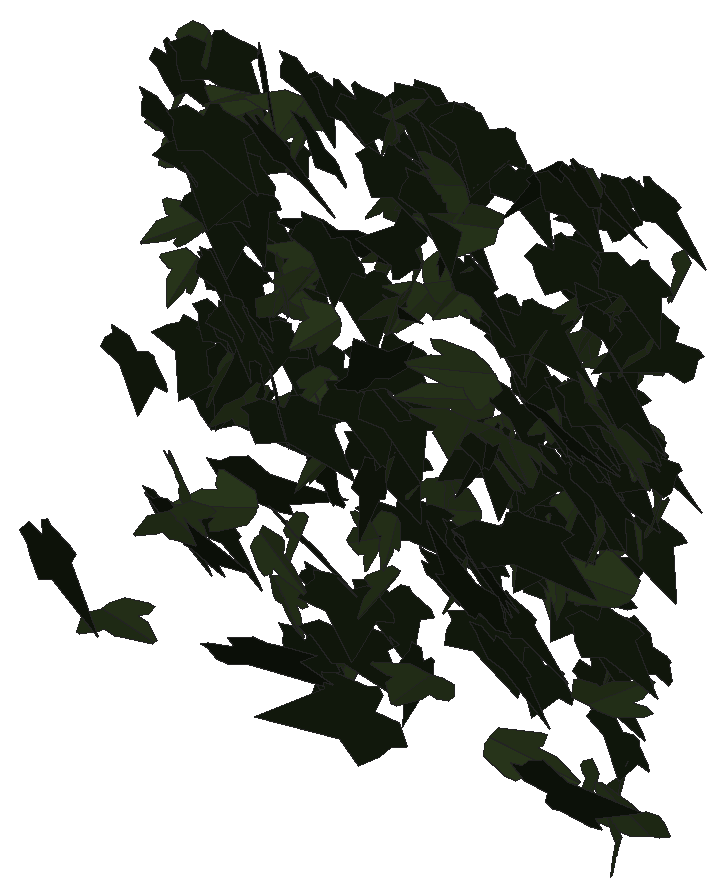
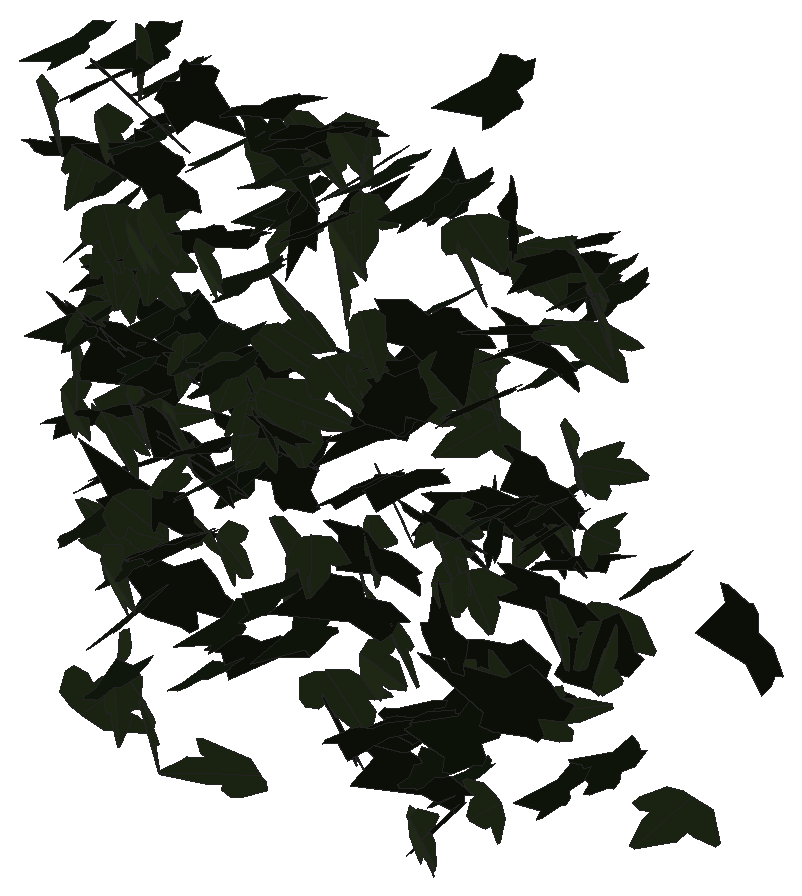
# SketchUp Ruby script. Lengths in millimetres.
U = 1.mm
M = Sketchup.active_model
def pt(a) = Geom::Point3d.new(a.map { |v| v * U })
def face(e, loops, mat)
  f = e.add_face(loops[0].map { |a| pt(a) })
  loops[1..].each { |l| e.add_face(l.map { |a| pt(a) }).erase! }
  f.material = f.back_material = mat if mat
  f
end
# faces: each face lists its corners as indices into pts; further lists are holes
def faces(e, pts, list, mat = nil) = list.each { |f| face(e, (f[0].is_a?(Array) ? f : [f]).map { |l| l.map { |i| pts[i] } }, mat) }
# xy, xz, yz: faces in a plane at the given z, y or x. An outline is a flat list of corners, or four numbers for a rectangle; further outlines are holes
def ring(l) = l.size == 4 ? [[l[0], l[1]], [l[2], l[1]], [l[2], l[3]], [l[0], l[3]]] : l.each_slice(2).to_a
def flat(e, list, mat, &to3) = list.each { |f| face(e, (f[0].is_a?(Array) ? f : [f]).map { |l| ring(l).map { |u, v| to3.(u, v) } }, mat) }
def xy(e, z, list, mat = nil) = flat(e, list, mat) { |x, y| [x, y, z] }
def xz(e, y, list, mat = nil) = flat(e, list, mat) { |x, z| [x, y, z] }
def yz(e, x, list, mat = nil) = flat(e, list, mat) { |y, z| [x, y, z] }
def lines(e, pts, list) = list.each { |a, b| e.add_line(pt(pts[a]), pt(pts[b])) }
# prism: a flat outline (further loops are holes) pulled along v
def prism(e, loops, v, mat = nil)
  f = face(e, loops, mat); d = Geom::Vector3d.new(v.map { |x| x * U })
  f.pushpull(f.normal.samedirection?(d) ? d.length : -d.length)
end
def box(e, o, s, mat = nil) = prism(e, [[o, [o[0] + s[0], o[1], o[2]], [o[0] + s[0], o[1] + s[1], o[2]], [o[0], o[1] + s[1], o[2]]]], [0, 0, s[2]], mat)
def at(x, y, z, deg = 0) = Geom::Transformation.translation(pt([x, y, z])) * Geom::Transformation.rotation(ORIGIN, Z_AXIS, deg.degrees)
def axes(o, x, y, z) = Geom::Transformation.new([*x, 0, *y, 0, *z, 0, *pt(o).to_a, 1])
def part(name) = M.definitions.add(name)
# library, detail: a bought-in or finely detailed component or shape, given as its bounding box
def library(name, o, s) = part(name).tap { |d| box(d.entities, o, s) }
def detail(e, o, s) = box(e.add_group.entities, o, s)
def put(e, d, t, mat = nil) = e.add_instance(d, t).tap { |i| i.material = mat if mat }
def group(e, t, mat = nil) = e.add_group.tap { |g| g.transformation = t; g.material = mat if mat }.entities
root = M.entities
M.materials.add("efeu1").color = [18, 25, 13]
M.materials.add("efeu2").color = [43, 57, 29]
c1 = part("ivyleaf_9")
p = [[39.1,54.8,31.7],[34.5,51.8,30.2],[-5.3,25.2,17.3],[-17.9,28.3,20.9],[-21.6,21.7,17],[-20.2,4.3,5.3],
  [-22.9,-0.3,2.5],[-17.1,-4,-0.6],[-2,-2.1,-1.2],[-0.7,-15.4,-10.1],[16.6,-22.3,-16.7],[21.1,-15.1,-12.5],
  [32.7,-10.7,-11],[46.1,-1.8,-6.6],[30.8,11.2,3.8]]
faces(c1.entities,p,[[0,1,2,3,4,5,6,7,8,9,10,11,12,13,14]],"efeu1")
c2 = part("ivyleaf_10")
p = [[0,12.8,-0.8],[-1.5,51.3,-10.9],[-4.9,51,-11.6],[-13.6,26.5,-7.3],[-13.2,15.9,-4.6],[-21.1,19.3,-7.2],
  [-29.5,16.3,-8.3],[-29.2,8.3,-6.2],[-19.7,-9.8,0.5],[-7.6,-13,4],[1,-12.2,5.8],[-0.4,51.1,-11.1],
  [-1.5,51.1,-10.9],[1,-12.4,5.9],[16.9,-12.4,3.5],[35.1,9.1,-5.1],[35,12.9,-6.1],[20.5,16.4,-4.9],
  [15.8,15,-3.8],[15.3,27.6,-7.1],[12.8,31.3,-7.8]]
faces(c2.entities,p,[[0,1,2,3,4,5,6,7,8,9,10],[11,12,0,13,14,15,16,17,18,19,20]],"efeu2")
put(root,c1,axes([3275.9,692.6,3007],[-0.14486,-1.00887,0.49826],[-0.08657,-0.49624,-1.01171],[2.13974,-0.08838,-0.0072]))
put(root,c2,axes([3286.5,780.7,3096],[-0.33808,-0.61445,0.90299],[0.50553,-0.91169,-0.56812],[2.01631,0.12555,0.29385]))
put(root,c2,axes([3301.5,765.3,3171.2],[-0.25019,-0.30689,1.0629],[-0.26477,-1.05729,-0.32247],[2.08882,-0.17078,0.08643]))
put(root,c2,axes([3304.1,758.5,3378.3],[0.77432,-1.06826,-0.1193],[-0.06905,0.11384,-1.14309],[2.04458,0.40842,0.00657]))
put(root,c2,axes([3293.5,619.6,2680.6],[-1.26151,-0.64825,-0.76951],[1.02479,0.54989,-0.92705],[1.61765,-0.85389,-0.01281]))
put(root,c1,axes([3291.1,739.6,3409.1],[1.17078,-0.84906,-0.46175],[-0.28698,0.45633,-1.03999],[1.81692,0.61919,0.13328]))
put(root,c2,axes([3313.1,769.7,3429.8],[1.35855,-0.89446,0.08275],[0.07875,-0.07284,-1.14431],[1.7078,0.7149,-0.01306]))
put(root,c1,axes([3291,733.8,2778.5],[0.69295,-0.95835,0.35796],[0.29917,-0.32303,-1.02473],[1.92388,0.39541,0.03042]))
put(root,c2,axes([3328.2,773.8,3202.9],[0.82032,-1.02813,-0.17206],[-0.06254,0.17269,-1.11424],[1.98297,0.43077,0.03603]))
put(root,c2,axes([3336.5,742.1,3322.4],[2.09345,0.29562,-0.47888],[-0.87545,-0.13347,-1.13896],[-0.61709,1.19224,-0.00877]))
put(root,c1,axes([3294.8,487.3,2842.9],[-0.34645,0.02579,-1.46881],[2.77466,-0.1788,-0.18382],[-0.34376,-1.46921,-0.00341]))
put(root,c1,axes([3315.4,707,3351.7],[0.28437,-1.09403,0.44387],[0.18712,-0.43433,-1.1036],[2.23919,0.17523,0.03585]))
put(root,c2,axes([3356.3,681.5,2852.6],[-1.21182,0.92811,0.25923],[0.26347,-0.21938,1.12549],[1.81496,0.65153,0.0097]))
put(root,c1,axes([3355.5,741,3025.6],[-1.17473,-0.89334,0.26512],[-0.13803,-0.27098,-1.08196],[1.76812,-0.61469,0.09168]))
put(root,c1,axes([3328.7,777.4,2758.8],[0.94761,-0.97704,0.03663],[-0.00417,-0.04222,-1.09639],[1.86081,0.49746,-0.02111]))
put(root,c2,axes([3361.6,755.7,2963.8],[1.14733,-0.73352,-0.57743],[-0.2711,0.60703,-0.91985],[1.75589,0.57302,0.23528]))
put(root,c1,axes([3333.7,765.3,3428.4],[0.05308,-0.87016,-0.75638],[0.24177,0.75431,-0.8631],[2.18092,-0.06244,0.11409]))
put(root,c1,axes([3352,775.6,3112],[0.06462,-1.06748,0.33836],[0.00337,-0.33846,-1.06798],[2.13123,0.0329,-0.00857]))
put(root,c2,axes([3396.3,740.1,2814.8],[-0.12103,0.24107,1.20612],[-0.6106,-1.16917,0.21677],[2.25985,-0.30299,0.12317]))
put(root,c1,axes([3362.7,750.6,3070.1],[0.49186,-1.0281,-0.34019],[-0.20326,0.32384,-1.05983],[2.05098,0.27865,-0.02345]))
put(root,c1,axes([3365.4,765.9,3134.4],[-0.71401,-0.16215,-1.07741],[2.0477,0.12445,-0.39338],[0.32682,-1.13405,0.11089]))
put(root,c2,axes([3411.7,730.2,3379.9],[-0.51329,-0.39232,1.1537],[-0.47853,-1.13827,-0.44586],[2.26929,-0.32877,0.16694]))
put(root,c2,axes([3410.2,739.2,3389.1],[-0.55097,-1.06706,0.39731],[-0.24254,-0.37701,-1.1054],[2.15342,-0.31548,-0.02285]))
put(root,c1,axes([3391,715.9,3237.1],[-0.29383,-1.07995,0.41912],[0.08629,-0.42813,-1.08648],[2.20303,-0.12727,0.09846]))
put(root,c1,axes([3424.4,789.5,3315.8],[-1.48506,-0.67046,0.46791],[-0.33759,-0.49258,-1.00161],[1.51898,-0.76496,0.23486]))
put(root,c2,axes([3415.1,690.3,3039.7],[0.56074,-1.08245,0.19778],[0.1243,-0.18718,-1.12175],[2.09053,0.30147,0.01365]))
put(root,c2,axes([3409.7,598.7,2867.3],[-1.25696,-0.83169,-0.62451],[0.72221,0.4961,-1.06198],[1.84298,-0.76164,-0.00977]))
put(root,c1,axes([3379.9,734.8,2971.8],[0.07238,-0.3789,-1.04799],[1.61338,0.69048,-0.21887],[1.37665,-0.78928,0.31161]))
put(root,c1,axes([3421.3,712.3,3034.7],[-1.77576,0.17916,-0.7124],[1.34266,-0.10242,-0.94973],[-0.38964,-1.16943,-0.02596]))
put(root,c1,axes([3397.4,676.3,3387.8],[0.2046,-1.03952,-0.5103],[0.23278,0.51982,-1.03315],[2.19161,0.04183,0.15737]))
put(root,c1,axes([3424.5,679.8,3342.1],[-1.59055,-0.86228,-0.29175],[0.36911,0.21831,-1.20076],[1.69271,-0.85784,-0.01231]))
put(root,c1,axes([3421.7,752.1,3077.9],[-0.6598,-1.12972,0.06879],[-0.02694,-0.06761,-1.1817],[2.1539,-0.34691,0.00629]))
put(root,c1,axes([3402.9,716.7,3277.6],[0.63442,-0.92086,-0.61342],[0.24397,0.66848,-0.93386],[2.09165,0.20133,0.29498]))
put(root,c1,axes([3385,767,2830.2],[0.54237,-0.16166,1.12772],[2.04029,-0.35534,-0.32184],[0.73376,1.10757,0.06135]))
put(root,c1,axes([3428.3,744.2,3077.5],[-1.5303,-0.63244,-0.46672],[0.68007,0.30056,-1.02289],[1.33241,-0.87978,-0.01395]))
put(root,c1,axes([3412.6,723.6,3275.1],[-1.04247,-0.26962,-1.00386],[1.95669,0.02656,-0.56811],[0.2913,-1.14327,0.22354]))
put(root,c1,axes([3394.1,630.3,2827.8],[0.40359,-0.54738,1.23379],[1.2456,-1.05059,-0.57859],[2.24669,0.68079,0.09914]))
put(root,c1,axes([3422.2,753.9,3441.3],[-0.00045,-0.08305,-1.23674],[2.08051,-0.58301,0.03894],[-1.11206,-1.0907,0.07335]))
put(root,c2,axes([3440.2,773.4,2699.9],[-1.17713,0.58485,-0.59444],[0.55905,-0.53987,-0.83678],[-1.48538,-0.66667,0.15614]))
put(root,c2,axes([3462.6,776.6,2972.4],[-0.58577,-1.0108,0.14745],[-0.0633,-0.144,-1.05657],[1.94308,-0.30941,0.01003]))
put(root,c2,axes([3459.2,673.1,3014],[-0.65671,-1.0191,-0.60265],[0.42266,0.56087,-1.0756],[2.21331,-0.40948,0.02659]))
put(root,c1,axes([3455.1,776.1,3050.6],[-0.01819,-1.06825,0.28735],[-0.04314,-0.28711,-1.06812],[2.10492,-0.01512,-0.01941]))
put(root,c2,axes([3483.9,749.3,3404.7],[-1.37082,-0.72825,0.49988],[-0.15183,-0.58873,-0.97265],[1.67423,-0.64966,0.32108]))
put(root,c1,axes([3460.4,757.2,3199.7],[0.39703,-1.05238,-0.35762],[-0.01324,0.36262,-1.07116],[2.11534,0.19979,0.06042]))
put(root,c2,axes([3481.4,763.7,3368.5],[1.07343,-0.9853,0.35993],[0.30266,-0.32362,-1.13511],[1.97335,0.5856,-0.02169]))
put(root,c1,axes([3449.1,784.4,2780.9],[1.23171,-0.92448,0.49192],[0.57851,-0.38755,-1.12823],[1.90724,0.71459,0.02453]))
put(root,c1,axes([3480.7,719.1,2985.3],[-0.07503,-0.04675,1.18196],[-0.25901,-1.17459,-0.05099],[2.23632,-0.13761,0.03375]))
put(root,c2,axes([3480,725.7,3144.8],[-1.13539,-0.49919,-0.8205],[1.19309,0.52937,-0.77787],[1.38479,-0.86537,-0.00254]))
put(root,c2,axes([3472.6,726.3,3185.1],[0.40074,-0.52441,1.07679],[1.43762,-0.7903,-0.53259],[1.76896,0.76107,0.1889]))
put(root,c2,axes([3494,739.4,2820.3],[1.00137,-0.98515,0.36041],[0.32473,-0.31747,-1.11685],[1.96989,0.55312,0.0009]))
put(root,c2,axes([3514,744,2995.5],[0.76936,-0.52426,-0.91045],[-0.57949,0.8752,-0.63915],[1.91371,0.47579,0.17248]))
put(root,c2,axes([3470.9,703,2801.5],[0.68061,-0.2319,1.0365],[1.85627,-0.36128,-0.41734],[0.80028,1.03522,0.08653]))
put(root,c2,axes([3513.9,720.3,3187.1],[-0.03865,-0.99944,0.55469],[0.00422,-0.55481,-0.99957],[2.17544,-0.01668,0.01179]))
put(root,c1,axes([3525.8,778.7,3036.4],[-2.0025,0.06643,-0.22014],[0.40903,-0.08246,-1.05212],[-0.1556,-1.07179,0.06731]))
put(root,c2,axes([3525,738.1,3214.5],[-1.19954,-0.84539,0.58403],[-0.22436,-0.62113,-1.02631],[1.94264,-0.59375,0.2421]))
put(root,c2,axes([3522.3,759,3010],[1.21978,-0.76042,-0.6346],[-0.44834,0.61715,-0.97742],[1.83089,0.65773,0.18344]))
put(root,c1,axes([3505.2,774,2870.8],[-0.77004,0.41446,0.94509],[0.11122,-1.00431,0.46544],[1.96091,0.21972,0.34474]))
put(root,c1,axes([3491.5,760.9,3442.9],[0.24518,-1.07402,0.41956],[0.16905,-0.41167,-1.0811],[2.18799,0.15216,0.03651]))
put(root,c2,axes([3524.1,755.9,3024.6],[0.70996,0.66662,-0.89608],[-0.76445,-0.80146,-0.76343],[-1.98336,0.54753,-0.02651]))
put(root,c1,axes([3511.6,783.6,2717.6],[-0.18946,-0.87645,0.59303],[0.28614,-0.60132,-0.86346],[1.99359,0.00302,0.18029]))
put(root,c2,axes([3536.1,782.3,2639.9],[0.31353,-0.9735,0.30647],[0.18502,-0.29406,-0.98633],[1.93358,0.18599,0.04469]))
put(root,c2,axes([3532.8,739.3,2931.9],[0.18324,-0.37219,1.11823],[0.51565,-1.08492,-0.38443],[2.18293,0.28752,-0.00306]))
put(root,c1,axes([3556.7,735.1,3258.2],[1.14723,0.64029,-0.79161],[-1.06393,-0.56074,-0.87923],[-1.61953,0.82193,0.01684]))
put(root,c1,axes([3515.6,687.4,3013.5],[-0.30611,-0.59584,-0.9611],[0.88164,0.85087,-0.60502],[1.9633,-0.47499,0.12184]))
put(root,c1,axes([3521.8,717.6,2674.3],[0.47576,-1.07113,0.17564],[0.07623,-0.17101,-1.09991],[2.06439,0.25317,0.00014]))
put(root,c1,axes([3526.2,770.3,3430.2],[0.92565,-1.04803,-0.04095],[-0.03017,0.03778,-1.15538],[1.9959,0.48662,0.00152]))
put(root,c1,axes([3552,749.3,2609.3],[-0.42825,-0.61711,0.98012],[-0.68291,-0.91218,-0.65671],[2.09586,-0.42332,-0.01371]))
put(root,c2,axes([3559.2,757,2622.2],[0.84709,-0.9799,0.09472],[0.07088,-0.08711,-1.07624],[1.87229,0.44664,-0.00211]))
put(root,c2,axes([3561.3,709.5,3142.3],[-0.41263,-0.17831,1.10809],[0.23387,-1.12556,-0.15708],[2.12321,0.08933,0.23265]))
put(root,c1,axes([3531.2,575.3,2733.7],[2.33724,0.44859,0.46219],[0.82097,0.16613,-1.3074],[-0.91032,1.30159,0.00758]))
put(root,c1,axes([3555,709.8,3387.3],[-0.5154,-0.4097,1.04657],[0.03984,-1.07817,-0.41666],[2.13865,-0.07865,0.25998]))
put(root,c1,axes([3564.1,713.6,3258.8],[-0.22224,-1.08771,0.36615],[-0.05125,-0.36534,-1.0939],[2.18367,-0.11928,0.01159]))
put(root,c1,axes([3570.4,744.9,2751.6],[-0.74218,-1.00944,-0.1488],[0.0883,0.14159,-1.08212],[1.93992,-0.39264,-0.00767]))
put(root,c1,axes([3556.7,746.2,2689.7],[-0.47229,-0.42512,-1.00772],[1.52611,0.63202,-0.46408],[1.4156,-0.82319,0.16411]))
put(root,c2,axes([3605.9,736.4,2845.3],[0.77468,-0.65288,-0.73768],[-0.66945,0.64924,-0.76869],[1.75126,0.53699,0.03247]))
put(root,c1,axes([3559,780.4,3158.5],[0.27928,-0.48156,1.01776],[1.17132,-0.82516,-0.47917],[1.79442,0.61358,0.15438]))
put(root,c1,axes([3588.1,746,3198.7],[-0.47145,-1.09137,-0.19604],[0.06104,0.19373,-1.11907],[2.10946,-0.24952,-0.01143]))
put(root,c1,axes([3566,577.8,3474.8],[1.57759,-1.0411,0.02855],[0.02869,-0.02449,-1.33078],[1.98195,0.82904,-0.00346]))
put(root,c1,axes([3584,745.2,3446.1],[1.20847,-0.82265,-0.53617],[-0.14164,0.59634,-1.00312],[1.86348,0.57882,0.27146]))
put(root,c2,axes([3616.4,773.8,3244.2],[-0.28966,-1.11281,-0.02709],[0.00417,0.02705,-1.12316],[2.11852,-0.15221,-0.00149]))
put(root,c1,axes([3599.5,734.8,3041.9],[-0.42208,-1.04022,-0.37124],[0.09346,0.36899,-1.06325],[2.09997,-0.2255,-0.0273]))
put(root,c1,axes([3602,781.7,2742.1],[-0.32059,-1.02661,-0.32116],[0.06367,0.31992,-1.04018],[2.04622,-0.1708,-0.01795]))
put(root,c2,axes([3635.5,738.1,2963.2],[0.10029,-1.05707,-0.36706],[0.0317,0.36817,-1.05787],[2.12942,0.0443,0.03303]))
put(root,c2,axes([3636.8,748.1,3183.6],[-0.41201,-1.11946,-0.14462],[0.04914,0.14231,-1.14019],[2.14769,-0.21801,-0.00165]))
put(root,c1,axes([3608.9,763,2961.2],[-1.00484,-0.28013,-0.95176],[1.73408,0.28975,-0.59072],[0.74724,-1.04912,0.09099]))
put(root,c2,axes([3635,738,2797.2],[0.17478,-0.82512,0.77525],[0.1598,-0.77069,-0.83021],[2.14883,0.12443,-0.00132]))
put(root,c1,axes([3633.9,713.6,3093.2],[0.96135,0.44437,1.07602],[-1.48693,-0.74017,0.67244],[1.64258,-0.93011,-0.02104]))
put(root,c2,axes([3652.7,785.1,3181.2],[-1.08923,-0.80064,0.53157],[-0.2556,-0.54599,-0.96695],[1.81109,-0.55858,0.18323]))
put(root,c1,axes([3618.2,747.8,3104.8],[0.38706,-0.97242,-0.72905],[-0.00474,0.73885,-0.98619],[2.31308,0.16424,0.11997]))
put(root,c1,axes([3629.4,761.2,3032.2],[-0.00068,-1.18226,-0.1288],[-0.03512,0.12879,-1.18212],[2.26312,0.00165,-0.01838]))
put(root,c2,axes([3649,725.4,3453.3],[0.47551,-0.9244,-0.61852],[0.21433,0.6517,-0.92849],[2.10593,0.1424,0.23416]))
put(root,c2,axes([3644,731.2,2876.6],[1.2739,-0.79193,0.26859],[0.38603,-0.18001,-1.03623],[1.544,0.6984,0.03747]))
put(root,c1,axes([3679.6,646.4,2664.4],[-0.1938,-0.7318,-1.20891],[-0.3472,-1.19509,0.73881],[-2.667,0.20876,-0.00833]))
put(root,c2,axes([3658.1,723.1,3357],[-0.23478,-1.1411,-0.43764],[0.20504,0.428,-1.14633],[2.31693,-0.15351,0.0571]))
put(root,c2,axes([3662.3,756,3462.8],[-0.05814,-1.09356,0.41182],[-0.0228,-0.41165,-1.09399],[2.22385,-0.03281,-0.00045]))
put(root,c2,axes([3664.3,759,3339],[0.32646,-1.09042,0.35447],[0.05607,-0.3541,-1.10356],[2.18147,0.17229,-0.02468]))
put(root,c1,axes([3659.6,679.5,2977.5],[-1.1605,0.22528,-0.94837],[1.61295,-0.43012,-0.64708],[-0.91651,-1.04221,0.06205]))
put(root,c1,axes([3637.7,756.6,2886.4],[-0.21305,-0.22365,-1.09413],[1.33142,0.84308,-0.24391],[1.65671,-0.7063,0.05531]))
put(root,c1,axes([3655.1,710,3404],[0.7819,-1.14036,-0.40828],[-0.21605,0.39297,-1.21185],[2.2951,0.4255,0.02502]))
put(root,c2,axes([3694.7,719.5,3265.8],[0.41284,-0.99031,-0.56397],[-0.11464,0.56333,-1.01236],[2.16594,0.21857,0.05392]))
put(root,c2,axes([3691.2,773.4,2936.2],[-0.69812,-1.00026,-0.15339],[0.30683,0.10331,-1.05922],[1.90136,-0.38394,0.11461]))
put(root,c1,axes([3679.4,791.4,3354.9],[-0.31496,-1.1053,0.19456],[-0.06719,-0.19144,-1.1176],[2.13489,-0.16909,-0.00647]))
put(root,c1,axes([3687.2,764.1,3466.8],[-1.02451,-1.01708,-0.1947],[0.1458,0.17972,-1.15064],[1.96546,-0.5435,-0.01613]))
put(root,c1,axes([3693.4,730.2,2700.9],[-1.30374,0.32815,-0.78247],[1.38351,-0.29168,-0.75874],[-0.83284,-0.99822,-0.03552]))
put(root,c1,axes([3709.2,693,3307.8],[-0.17298,-0.11257,1.15808],[-1.38709,-0.89998,-0.14468],[1.7262,-0.73447,-0.00021]))
put(root,c1,axes([3693.2,783.2,3461.6],[-0.71791,-1.08245,0.13515],[-0.00221,-0.1426,-1.14539],[2.07611,-0.37446,0.04551]))
put(root,c2,axes([3731.4,686.2,2712.2],[-1.57654,-0.49623,0.46274],[-0.73353,-0.25688,-0.96541],[1.06277,-0.91341,0.02011]))
put(root,c2,axes([3680.6,779.4,3212.7],[1.18051,-0.5236,-0.82353],[1.25025,-0.49759,0.81115],[-1.37351,-0.90297,0.03054]))
put(root,c1,axes([3694.3,753.4,2828],[1.56585,-0.5227,-0.42626],[-0.40006,0.44016,-0.94546],[1.21972,0.8154,0.23712]))
put(root,c2,axes([3758.5,744.7,3091.1],[-0.5753,-0.1415,1.10941],[-1.61612,-0.71885,-0.32306],[1.38521,-0.89745,0.08385]))
put(root,c2,axes([3750.7,753.5,2927.7],[0.71864,-0.60551,-0.88548],[-0.8647,0.7601,-0.71352],[1.84943,0.59067,0.01046]))
put(root,c1,axes([3748.7,716.8,3324.6],[-0.0185,-0.02449,-1.21503],[-1.57295,0.89096,-0.01135],[1.69571,0.82619,-0.02378]))
put(root,c2,axes([3762.5,702,3413.2],[1.13364,-0.50535,-0.9431],[-1.19315,0.70986,-0.77632],[1.65017,0.86042,0.08657]))
put(root,c1,axes([3727.7,782.8,3396.3],[-0.55942,-1.03678,0.40255],[0.27697,-0.44865,-1.04923],[2.09851,-0.21717,0.2458]))
put(root,c2,axes([3781,725.2,3145.5],[1.11526,-0.20604,-1.04989],[-1.91764,0.29634,-0.62054],[0.68487,1.16527,-0.02783]))
put(root,c1,axes([3724.4,745,3352.3],[0.78186,-1.08714,-0.00895],[-0.00238,0.00909,-1.16217],[2.06911,0.41081,0.00204]))
put(root,c2,axes([3770.8,723.8,3065.9],[-2.04754,-0.43705,0.30582],[-0.53899,-0.11542,-1.16123],[0.86031,-1.11249,0.00034]))
put(root,c1,axes([3733.6,780.3,2862.2],[0.42705,-1.14973,0.31375],[0.13511,-0.3058,-1.17138],[2.26416,0.2351,0.01072]))
put(root,c1,axes([3741.9,701.2,3387.6],[0.00309,-1.22118,0.35141],[-0.04202,-0.35139,-1.22099],[2.41811,-0.00454,-0.02166]))
put(root,c1,axes([3786.4,730.9,3417.5],[-0.62374,1.08765,-0.05036],[-0.03973,-0.05886,-1.13536],[-2.07186,-0.32631,0.03693]))
put(root,c2,axes([3804.6,711.4,3362.8],[-0.3801,-0.14993,-1.19861],[-1.70562,-0.79619,0.24892],[-1.54147,0.91795,0.02013]))
put(root,c1,axes([3772.7,760.5,3465.3],[-0.89811,-1.03697,0.14446],[-0.07462,-0.14084,-1.13907],[1.99121,-0.47299,0.02247]))
put(root,c2,axes([3783.8,691.2,2863.5],[0.03969,-0.79247,-0.83201],[0.06721,0.83219,-0.79176],[2.18578,-0.0112,0.03945]))
put(root,c2,axes([3790,704.7,3278.3],[0.21951,0.48889,-1.11409],[-0.67747,-1.05655,-0.5005],[-2.21418,0.37174,0.04269]))
put(root,c1,axes([3812,745.9,3043.1],[-2.01428,-0.24788,0.07643],[-0.13696,-0.0279,-1.08696],[0.47431,-1.06076,0.01073]))
put(root,c1,axes([3782.1,753.1,2776.9],[-0.49324,-0.93451,-0.53693],[0.22589,0.52413,-0.96952],[2.03875,-0.28416,-0.02248]))
put(root,c2,axes([3795.3,758.3,3065],[-0.38305,-1.05471,-0.20418],[0.58749,0.1422,-1.0388],[1.95837,-0.24896,0.27169]))
put(root,c1,axes([3810.5,724.3,3058.9],[-1.32655,0.55547,-0.75282],[1.13471,-0.45973,-0.89123],[-1.37218,-0.91717,-0.00921]))
put(root,c2,axes([3801.6,729.8,3023.5],[-1.56895,0.68978,-0.18309],[0.22167,-0.14595,-1.07427],[-1.34004,-0.83176,0.03666]))
put(root,c2,axes([3833.8,745.8,2880.1],[0.115,0.10332,-1.13934],[-0.94775,1.02955,0.06695],[1.9602,0.49172,0.09922]))
put(root,c1,axes([3795.3,752.1,3237.3],[-0.04525,-1.11262,0.11863],[0.00745,-0.11873,-1.11286],[2.12953,-0.02323,0.00641]))
put(root,c1,axes([3787.4,700.6,3304.4],[0.86575,-1.07791,-0.02188],[-0.01531,0.02035,-1.16996],[2.05184,0.45496,0.0005]))
put(root,c1,axes([3806,735.8,3031.8],[-0.07815,-1.05748,0.55553],[-0.09173,-0.55394,-1.05802],[2.27156,-0.05875,-0.02361]))
put(root,c1,axes([3801.6,743.3,3223.4],[0.27251,-1.07328,0.22477],[0.15119,-0.21593,-1.08168],[2.0815,0.1562,0.04914]))
put(root,c1,axes([3809.2,788.5,3153.2],[-0.39081,-0.8747,0.65751],[0.15676,-0.67944,-0.87816],[2.0767,-0.11332,0.19002]))
put(root,c1,axes([3803.7,780.9,3406.1],[0.35191,-1.14119,-0.0532],[0.04808,0.05796,-1.15557],[2.17375,0.18347,0.03417]))
put(root,c1,axes([3800.6,767.2,2802.4],[1.195,-0.97333,-0.18569],[-0.12271,0.17924,-1.1575],[1.88185,0.62977,0.04244]))
put(root,c1,axes([3838.4,790.5,2969.2],[-0.80099,-0.71799,0.81878],[-0.40351,-0.80699,-0.81662],[2.03292,-0.44307,0.16052]))
put(root,c2,axes([3803.7,761.7,2607.5],[0.65305,0.26632,1.05489],[1.64579,0.60449,-0.43389],[-1.2566,0.93012,-0.02006]))
put(root,c1,axes([3843.6,783.6,3017.2],[-0.83448,-0.9341,0.34741],[-0.18962,-0.33655,-1.03067],[1.88725,-0.44684,0.05005]))
put(root,c1,axes([3826.8,758.3,3097.7],[0.08329,-1.03229,0.49712],[0.15564,-0.4934,-1.03176],[2.17504,0.07484,0.0548]))
put(root,c1,axes([3840.4,784.5,2724.7],[-0.50591,-0.89868,0.57094],[-0.02556,-0.58559,-0.92799],[2.02619,-0.23178,0.13085]))
put(root,c1,axes([3871.9,616.8,2892.5],[0.83933,-0.68015,1.07494],[-0.85369,0.98148,0.80504],[-2.26546,-0.62184,0.09489]))
put(root,c2,axes([3859.6,705.1,3077.1],[-2.03443,0.26006,-0.05666],[0.10358,-0.01599,-1.10013],[-0.49585,-1.07033,0.00267]))
put(root,c1,axes([3843.9,768.4,3127.9],[0.34015,-1.05558,0.29703],[0.16741,-0.28618,-1.06995],[2.08028,0.19563,0.03753]))
put(root,c1,axes([3887,758.4,3449.8],[-0.56859,0.50255,-0.98464],[0.58966,-0.94102,-0.57429],[-2.01961,-0.41623,0.10954]))
put(root,c2,axes([3877.7,733.7,3221.9],[0.70885,-0.95639,0.50622],[0.32927,-0.47585,-1.0263],[2.03296,0.41055,-0.01028]))
put(root,c1,axes([3875.6,607,2967.4],[2.00113,-0.34811,-0.7649],[-1.39063,0.22656,-1.10752],[0.79016,1.28035,-0.01199]))
put(root,c1,axes([3862.5,717.7,3252.3],[0.30908,-0.87289,-0.80503],[0.40643,0.82075,-0.84685],[2.22309,-0.02869,0.26674]))
put(root,c2,axes([3888.5,751.9,3111.7],[-0.25853,-1.08628,-0.14102],[0.4362,0.11077,-1.07403],[2.03861,-0.16146,0.21192]))
put(root,c1,axes([3910.8,722.6,2959.3],[-2.01768,0.03656,-0.45138],[0.85509,-0.05907,-1.06003],[-0.108,-1.15073,0.04007]))
put(root,c1,axes([3886.1,771.6,2873.5],[-0.13413,-1.17215,-0.15641],[0.08329,0.15399,-1.17377],[2.24906,-0.07561,0.03414]))
put(root,c2,axes([3888.9,744.2,2895],[1.6722,-0.57215,0.47806],[0.73991,-0.27889,-1.04831],[1.21082,0.96059,-0.01961]))
put(root,c2,axes([3909.7,766.1,2937.3],[-0.20098,0.91491,0.6919],[0.16293,-0.6866,0.92097],[2.17702,0.13585,-0.00505]))
put(root,c1,axes([3913.3,771.7,2860.2],[-0.85704,-0.87896,0.52011],[-0.27855,-0.50702,-0.98355],[1.9237,-0.46501,0.0893]))
put(root,c2,axes([3920.7,767.5,3275.5],[-0.13159,-1.0809,0.28869],[-0.02875,-0.28831,-1.08311],[2.12909,-0.0707,0.00322]))
put(root,c2,axes([3923.4,766.2,3230.6],[-0.80236,-1.02733,-0.34535],[0.22706,0.32432,-1.1104],[2.0502,-0.43797,-0.01218]))
put(root,c2,axes([3923.4,731.6,2998.7],[1.09841,-0.9261,-0.01061],[-0.03329,0.0016,-1.09113],[1.76235,0.57724,-0.014]))
put(root,c1,axes([3905.5,756.3,3146.7],[0.91125,-1.06287,-0.04257],[-0.02873,0.03989,-1.16573],[2.02428,0.47903,0.00262]))
put(root,c1,axes([3909.3,739.5,3444.3],[0.60036,-1.09083,-0.13741],[-0.02809,0.13874,-1.13527],[2.09228,0.31487,0.02419]))
put(root,c2,axes([3934.5,779.6,3254.1],[0.4712,-1.04968,0.41802],[0.11535,-0.41498,-1.07796],[2.14725,0.25264,-0.03382]))
put(root,c1,axes([3894.4,726.4,3109.6],[0.80436,-0.62187,0.88306],[1.07944,-0.6792,-0.74976],[1.74931,0.70505,0.05661]))
put(root,c2,axes([3972.8,716.2,3173.2],[-0.86843,0.15198,1.0031],[-1.80075,0.33321,-0.48089],[-0.69688,-1.05043,-0.00742]))
put(root,c1,axes([3915.5,770.5,3099.6],[0.6374,-1.09702,0.0499],[0.00125,-0.05197,-1.14691],[2.09001,0.33459,-0.01453]))
put(root,c1,axes([3916.1,738.1,3052],[0.3717,-1.08259,0.29529],[0.16499,-0.28428,-1.09955],[2.12928,0.21101,0.03365]))
put(root,c2,axes([3950.2,780.9,2901.8],[-0.64714,-0.73045,0.74123],[-0.10949,-0.76541,-0.78067],[1.97757,-0.28141,0.19934]))
put(root,c1,axes([3971.6,779.9,3118],[-2.09759,-0.03137,0.15529],[-0.29392,-0.03066,-1.10228],[0.06723,-1.1126,0.026]))
put(root,c2,axes([3948.7,746,2621.3],[0.78373,-0.96484,-0.33883],[-0.11706,0.34124,-1.04646],[1.94271,0.4098,0.07364]))
put(root,c1,axes([3928.5,724.2,2982.8],[-1.25217,-0.17528,-0.89599],[1.69721,0.11328,-0.67699],[0.37234,-1.10582,0.07267]))
put(root,c1,axes([3921.8,593.4,2866.8],[0.93991,-1.12594,0.3271],[0.21149,-0.30839,-1.2293],[2.22145,0.50575,-0.02137]))
put(root,c1,axes([3931.7,698.4,3376.3],[0.66065,-0.861,-0.7275],[-0.12632,0.74428,-0.91253],[2.14156,0.30951,0.1706]))
put(root,c1,axes([3925,758.5,2886.9],[-0.67118,0.21256,1.08646],[1.68619,-0.62951,0.41075],[1.26334,0.95314,0.02899]))
put(root,c1,axes([3910.3,749.1,3323.5],[0.60115,-0.07332,-1.13873],[2.06304,0.38837,0.27567],[0.67839,-1.11608,0.17074]))
put(root,c1,axes([3988.9,766.4,3430.3],[-1.72731,0.67082,0.127],[-0.185,0.08215,-1.12856],[-1.28614,-0.91274,-0.00823]))
put(root,c1,axes([3931.7,598.5,3030.7],[-0.34788,-0.35002,-1.29683],[1.02713,1.17936,-0.39438],[2.34102,-0.56946,-0.01967]))
put(root,c1,axes([3944.3,755.9,2767.9],[0.97968,-0.89841,-0.5316],[-0.47345,0.47007,-1.0353],[1.92952,0.57149,0.01588]))
put(root,c1,axes([3957.6,752.1,3346.8],[-0.79304,-0.81394,0.69371],[-0.04232,-0.73775,-0.87897],[2.03494,-0.33255,0.25206]))
put(root,c1,axes([3936.1,736.7,3471.5],[1.36821,-0.87906,-0.16659],[-0.01892,0.20585,-1.12909],[1.7027,0.70866,0.12132]))
put(root,c2,axes([3971,728.8,3463.7],[0.9169,-0.88599,-0.61923],[0.01935,0.68163,-0.96737],[2.05715,0.38849,0.2851]))
put(root,c2,axes([3967.2,743.7,3007.4],[0.87215,-0.95431,0.27283],[0.29322,-0.22847,-1.05793],[1.86612,0.4819,0.03872]))
put(root,c1,axes([3955.2,762.5,2814.1],[0.28506,-1.03675,0.23126],[0.10162,-0.22591,-1.04732],[2.01907,0.15774,0.02006]))
put(root,c1,axes([3963.5,786.2,2673.2],[-0.29049,-0.82463,0.67572],[0.00736,-0.68304,-0.83268],[2.02903,-0.11558,0.09976]))
put(root,c2,axes([3973.9,775.7,2810.3],[0.85443,-1.04275,0.49477],[0.30669,-0.46906,-1.13477],[2.17512,0.47575,-0.03436]))
put(root,c2,axes([3986,760.4,2985.2],[1.65878,-0.60712,-0.24728],[-0.31801,0.19205,-1.06046],[1.20643,0.88538,0.06046]))
put(root,c1,axes([3954.2,751.9,3075.6],[-0.70851,-0.2823,-1.06531],[1.71487,0.5695,-0.46578],[1.20773,-0.97424,0.03641]))
put(root,c2,axes([3991.3,743.9,2637.6],[-0.12119,-1.02531,-0.41092],[0.05217,0.41001,-1.02729],[2.10161,-0.0693,0.00181]))
put(root,c2,axes([3994.4,748.2,3193.6],[-0.55337,-1.12264,-0.1951],[0.10412,0.18737,-1.15967],[2.16614,-0.2958,0.0059]))
put(root,c2,axes([4001.2,747.7,3233.9],[-0.85878,-1.0268,0.03467],[-0.02873,-0.03123,-1.12157],[1.9551,-0.45148,-0.00125]))
put(root,c1,axes([3971.1,730.5,3181.2],[0.16559,-0.92088,-0.7029],[0.41938,0.70517,-0.89658],[2.16459,-0.06618,0.22748]))
put(root,c2,axes([4029.5,683.3,2947.2],[0.51708,0.35664,1.17355],[-1.45766,-0.88952,0.44764],[1.82331,-0.81227,0.02506]))
put(root,c2,axes([4039.1,726,2595.3],[-1.85675,0.00171,-0.57933],[-1.10113,-0.06107,0.97413],[-0.05655,1.13299,0.05338]))
put(root,c1,axes([3993.3,735.6,3281.3],[0.11044,-1.11771,0.36298],[0.10978,-0.36028,-1.1186],[2.23389,0.07296,0.03703]))
put(root,c2,axes([4019,730.1,3337.9],[0.27331,-1.16815,0.11398],[0.03305,-0.11271,-1.17694],[2.23354,0.14461,0.00347]))
put(root,c2,axes([4020.7,669.2,3023],[0.4944,-1.00547,-0.38903],[-0.02533,0.39714,-1.03533],[2.0517,0.24719,0.08096]))
put(root,c2,axes([4015.4,772.4,3115.7],[-0.62407,-0.75345,0.73683],[0.5509,-0.80639,-0.69576],[1.92856,-0.01346,0.43718]))
put(root,c1,axes([4046.4,753.4,3103.9],[-2.11484,0.34098,-0.19346],[0.354,-0.0533,-1.16233],[-0.6568,-1.12666,-0.00356]))
put(root,c2,axes([4011.2,716.9,3139.4],[-1.5661,0.68314,-0.46626],[0.67014,-0.3058,-1.06945],[-1.42436,-0.895,0.00951]))
put(root,c1,axes([4004.3,761.8,2995.6],[-0.10553,-1.12464,-0.42776],[0.27425,0.41893,-1.12009],[2.27352,-0.10274,0.11526]))
put(root,c2,axes([4025.1,784.7,3011.8],[0.36868,-0.98876,0.41748],[0.26179,-0.39785,-1.0061],[2.02581,0.23136,0.05404]))
put(root,c1,axes([4029.8,759.6,2829.4],[-0.78409,-0.54548,0.85973],[-0.25466,-0.89039,-0.62906],[1.92098,-0.34069,0.26752]))
put(root,c1,axes([4018.7,701.3,3220.1],[1.19024,-0.87453,-0.61668],[-0.68566,0.50051,-1.07513],[1.91771,0.72174,-0.00166]))
put(root,c1,axes([4007.5,769.8,3110],[1.18108,-0.92662,0.00007],[0.08409,0.02951,-1.11397],[1.76154,0.61987,0.05313]))
put(root,c2,axes([4017.9,680.4,2783.8],[-1.21672,-0.65848,0.65321],[0.88262,0.46012,0.91772],[-1.52875,0.78973,0.00996]))
put(root,c1,axes([4013.5,681.9,2891.1],[0.5306,-1.02264,-0.48464],[0.07878,0.50801,-1.04814],[2.15235,0.23351,0.15784]))
put(root,c1,axes([3997.8,604.7,2680.8],[0.28647,-0.24375,1.19736],[1.83022,-0.72066,-0.26759],[1.43474,0.96797,0.10228]))
put(root,c1,axes([4016.3,769.5,3462.5],[0.97646,-1.04605,-0.1518],[0.04988,0.18128,-1.16058],[2.01107,0.5034,0.10249]))
put(root,c2,axes([4051.9,743.1,3049.1],[0.5771,-0.92257,-0.63701],[-0.05311,0.65348,-0.95971],[2.13306,0.26587,0.14845]))
put(root,c1,axes([4036.6,714.9,3382.2],[0.11349,-1.16155,-0.10993],[-0.01209,0.10975,-1.16308],[2.2205,0.05996,-0.00071]))
put(root,c1,axes([4033.7,653.2,3105.7],[0.20082,-1.03428,0.57558],[0.30006,-0.56044,-1.03596],[2.23265,0.16835,0.08745]))
put(root,c2,axes([4064.9,642,2622.3],[0.53568,-0.57133,-1.07538],[-0.08933,1.09782,-0.59554],[2.31586,0.1745,0.22578]))
put(root,c2,axes([4059.1,714.4,3276.1],[-0.47625,-0.9226,-0.63681],[0.41275,0.60032,-0.95495],[2.09325,-0.32828,0.04341]))
put(root,c1,axes([4086.5,730,3291.5],[-1.90641,-0.40724,0.33238],[-0.53624,-0.1879,-1.07935],[0.84458,-1.03853,0.06495]))
put(root,c2,axes([4073.8,767.3,3373.2],[0.77756,-1.07903,-0.22505],[-0.08162,0.22427,-1.15314],[2.09621,0.40898,0.03858]))
